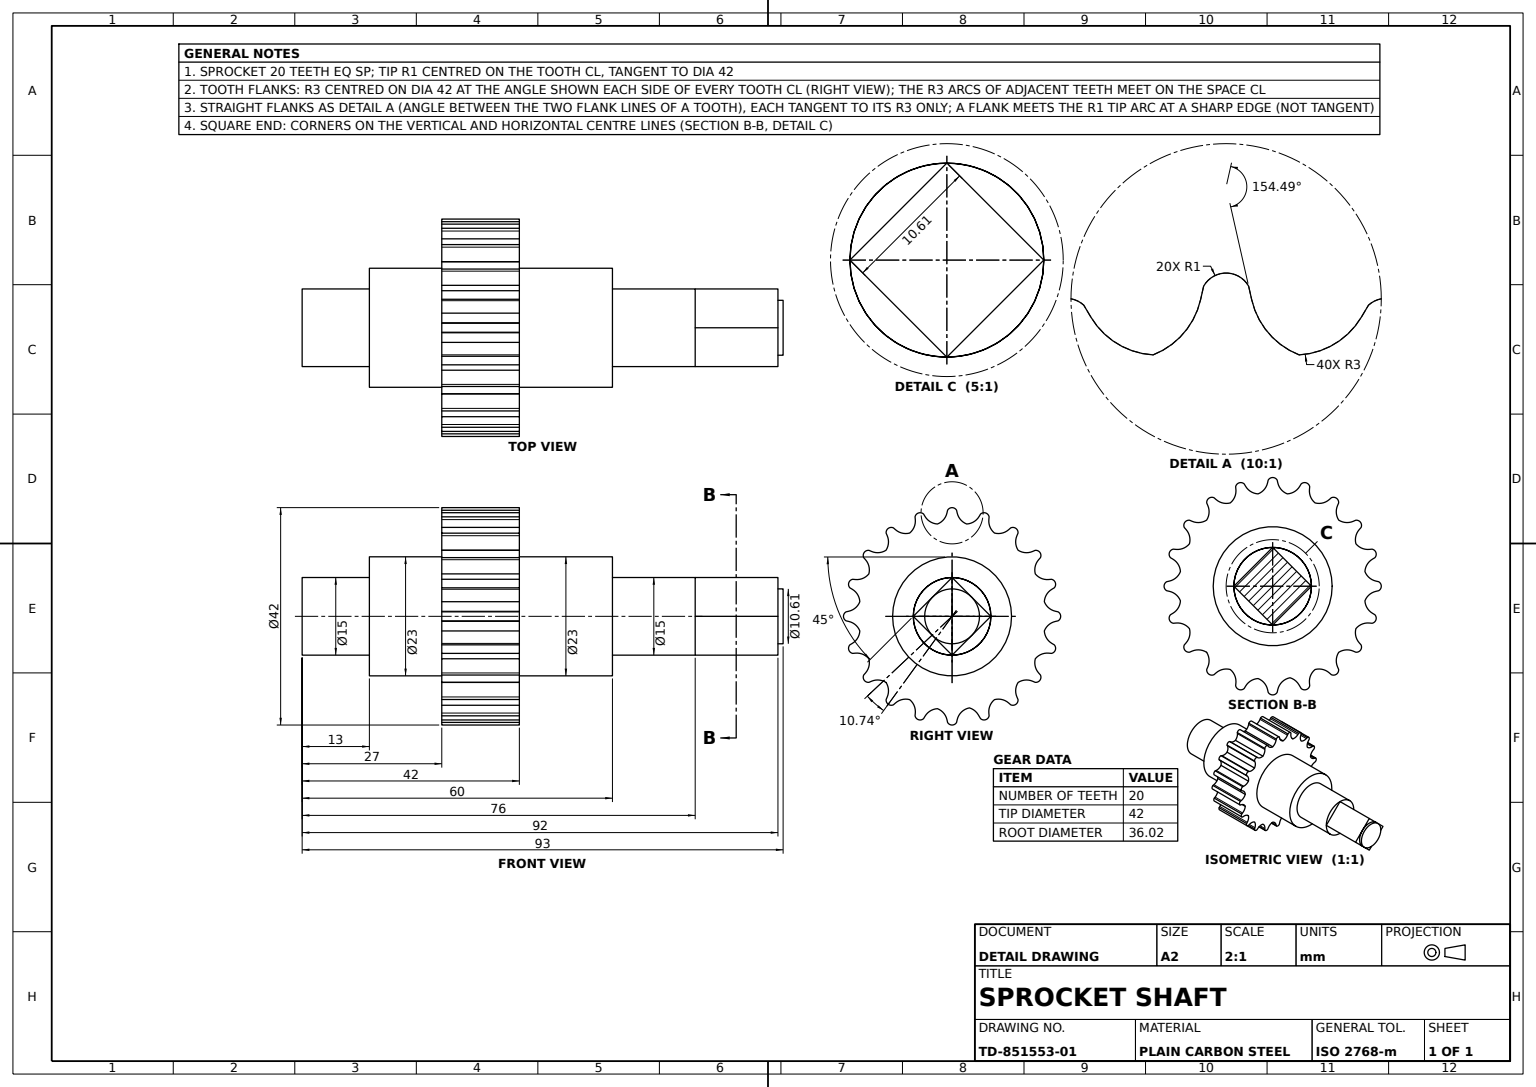
solid
v1 (12.755705,-16.18034,25.5)
v2 (12.749422,-16.068415,25.5)
e1 v1 v2 CIRCLE(AX(P(11.755705,-16.18034,25.5),D(0,0,1),D(-0.951056516,-0.309016994,0)),1)
v3 (12.755705,-16.18034,10.5)
e2 v3 v1 LINE
v4 (12.749422,-16.068415,10.5)
e3 v3 v4 CIRCLE(AX(P(11.755705,-16.18034,10.5),D(0,0,1),D(-0.951056516,-0.309016994,0)),1)
e4 v4 v2 LINE
face CYL(AX(P(11.755705,-16.18034,10.5),D(0,0,1),D(1,0,0)),1) [-e1 -e2 e3 e4]
v5 (-11.5,0,-7.5)
v6 (11.5,0,-7.5)
e5 v5 v6 CIRCLE(AX(P(0,0,-7.5),D(0,0,-1),D(-1,0,0)),11.5)
e6 v6 v5 CIRCLE(AX(P(0,0,-7.5),D(0,0,-1),D(-1,0,0)),11.5)
v7 (-7.5,0,-7.5)
v8 (7.5,0,-7.5)
e7 v7 v8 CIRCLE(AX(P(0,0,-7.5),D(0,0,-1),D(-1,0,0)),7.5)
e8 v8 v7 CIRCLE(AX(P(0,0,-7.5),D(0,0,-1),D(-1,0,0)),7.5)
face PLANE(AX(P(0,7.5,-7.5),D(0,0,-1),D(-1,0,0))) [e5 e6] [-e7 -e8]
v9 (3.75,3.75,-39.5)
v10 (5.303301,0,-39.5)
e9 v9 v10 CIRCLE(AX(P(0,0,-39.5),D(0,0,-1),D(-1,0,0)),5.303301)
v11 (7.5,0,-39.5)
e10 v9 v11 LINE
v12 (3.75,-3.75,-39.5)
e11 v11 v12 LINE
e12 v10 v12 CIRCLE(AX(P(0,0,-39.5),D(0,0,-1),D(-1,0,0)),5.303301)
face PLANE(AX(P(0,0,-39.5),D(0,0,-1),D(-1,0,0))) [-e9 e10 e11 -e12]
v13 (-16.090715,8.198629,10.5)
v14 (-16.736721,10.938339,10.5)
e13 v13 v14 CIRCLE(AX(P(-18.992374,8.960454,10.5),D(0,0,1),D(-1,0,0)),3)
v15 (-16.090715,8.198629,25.5)
e14 v15 v13 LINE
v16 (-16.736721,10.938339,25.5)
e15 v16 v15 CIRCLE(AX(P(-18.992374,8.960454,25.5),D(0,0,-1),D(1,0,0)),3)
e16 v14 v16 LINE
face CYL(AX(P(-18.992374,8.960454,0),D(0,0,-1),D(-1,0,0)),3) rev [-e13 -e14 -e15 -e16]
v17 (-17.090834,-11.342183,25.5)
v18 (-16.068415,-12.749422,25.5)
e17 v17 v18 CIRCLE(AX(P(-16.18034,-11.755705,25.5),D(0,0,1),D(-0.309016994,0.951056516,0)),1)
v19 (-17.090834,-11.342183,10.5)
e18 v19 v17 LINE
v20 (-16.068415,-12.749422,10.5)
e19 v19 v20 CIRCLE(AX(P(-16.18034,-11.755705,10.5),D(0,0,1),D(-0.309016994,0.951056516,0)),1)
e20 v20 v18 LINE
face CYL(AX(P(-16.18034,-11.755705,10.5),D(0,0,1),D(1,0,0)),1) [-e17 -e18 e19 e20]
v21 (-19.2977,-5.231047,25.5)
v22 (-19.2977,-5.231047,10.5)
e21 v21 v22 LINE
v23 (-19.759276,-5.505699,10.5)
e22 v22 v23 LINE
v24 (-19.759276,-5.505699,25.5)
e23 v23 v24 LINE
e24 v21 v24 LINE
face PLANE(AX(P(-2.747228,4.616964,10.5),D(-0.511351213,0.859371827,0),D(-0.859371827,-0.511351213,0))) [e21 e22 e23 -e24]
v25 (-8.198629,-16.090715,10.5)
v26 (-10.938339,-16.736721,10.5)
e25 v25 v26 CIRCLE(AX(P(-8.960454,-18.992374,10.5),D(0,0,1),D(-1,0,0)),3)
v27 (-8.198629,-16.090715,25.5)
e26 v27 v25 LINE
v28 (-10.938339,-16.736721,25.5)
e27 v28 v27 CIRCLE(AX(P(-8.960454,-18.992374,25.5),D(0,0,-1),D(1,0,0)),3)
e28 v26 v28 LINE
face CYL(AX(P(-8.960454,-18.992374,0),D(0,0,-1),D(-1,0,0)),3) rev [-e25 -e26 -e27 -e28]
v29 (-3.75,-3.75,-39.5)
v30 (-7.5,0,-39.5)
e29 v29 v30 LINE
v31 (0,-7.5,-39.5)
e30 v31 v29 LINE
v32 (0,-7.5,-23.5)
e31 v32 v31 LINE
v33 (-7.5,0,-23.5)
e32 v32 v33 LINE
e33 v33 v30 LINE
face PLANE(AX(P(-3.75,-3.75,-23.5),D(-0.707106781,-0.707106781,0),D(0.707106781,-0.707106781,0))) [-e29 -e30 -e31 e32 e33]
v34 (0.869722,20.493543,10.5)
v35 (0.869722,20.493543,25.5)
e34 v34 v35 LINE
v36 (-0.869722,20.493543,10.5)
e35 v34 v36 CIRCLE(AX(P(0,20,10.5),D(0,0,1),D(0.951056516,-0.309016994,0)),1)
v37 (-0.869722,20.493543,25.5)
e36 v36 v37 LINE
e37 v35 v37 CIRCLE(AX(P(0,20,25.5),D(0,0,1),D(0.951056516,-0.309016994,0)),1)
face CYL(AX(P(0,20,10.5),D(0,0,1),D(1,0,0)),1) [-e34 e35 e36 -e37]
v38 (17.18034,-11.755705,10.5)
v39 (17.090834,-11.342183,10.5)
e38 v38 v39 CIRCLE(AX(P(16.18034,-11.755705,10.5),D(0,0,1),D(-0.809016994,-0.587785252,0)),1)
v40 (17.090834,-11.342183,25.5)
e39 v39 v40 LINE
v41 (17.18034,-11.755705,25.5)
e40 v41 v40 CIRCLE(AX(P(16.18034,-11.755705,25.5),D(0,0,1),D(-0.809016994,-0.587785252,0)),1)
e41 v38 v41 LINE
face CYL(AX(P(16.18034,-11.755705,10.5),D(0,0,1),D(1,0,0)),1) [e38 e39 -e40 -e41]
v42 (17.836695,2.825055,10.5)
v43 (17.836695,2.825055,25.5)
e42 v42 v43 LINE
v44 (19.2977,5.231047,10.5)
e43 v44 v42 CIRCLE(AX(P(20.831753,2.652932,10.5),D(0,0,1),D(-1,0,0)),3)
v45 (19.2977,5.231047,25.5)
e44 v45 v44 LINE
e45 v43 v45 CIRCLE(AX(P(20.831753,2.652932,25.5),D(0,0,-1),D(1,0,0)),3)
face CYL(AX(P(20.831753,2.652932,0),D(0,0,-1),D(-1,0,0)),3) rev [-e42 -e43 -e44 -e45]
v46 (-12.769664,-12.769664,25.5)
v47 (-12.537435,-15.57491,25.5)
e46 v46 v47 CIRCLE(AX(P(-15.293888,-14.390864,25.5),D(0,0,-1),D(1,0,0)),3)
v48 (-12.749422,-16.068415,25.5)
e47 v47 v48 LINE
v49 (-11.342183,-17.090834,25.5)
e48 v48 v49 CIRCLE(AX(P(-11.755705,-16.18034,25.5),D(0,0,1),D(-0.587785252,0.809016994,0)),1)
e49 v28 v49 LINE
v50 (-7.110897,-18.6869,25.5)
e50 v27 v50 CIRCLE(AX(P(-10.098331,-18.412597,25.5),D(0,0,-1),D(1,0,0)),3)
v51 (-7.160007,-19.221758,25.5)
e51 v50 v51 LINE
v52 (-5.505699,-19.759276,25.5)
e52 v51 v52 CIRCLE(AX(P(-6.18034,-19.02113,25.5),D(0,0,1),D(-0.809016994,0.587785252,0)),1)
v53 (-5.067521,-19.02288,25.5)
e53 v53 v52 LINE
v54 (-3.355095,-17.684551,25.5)
e54 v53 v54 CIRCLE(AX(P(-2.489406,-20.556933,25.5),D(0,0,-1),D(1,0,0)),3)
v55 (-0.988296,-19.969686,25.5)
e55 v54 v55 CIRCLE(AX(P(-3.914278,-20.631976,25.5),D(0,0,-1),D(1,0,0)),3)
v56 (-0.869722,-20.493543,25.5)
e56 v55 v56 LINE
v57 (0.869722,-20.493543,25.5)
e57 v56 v57 CIRCLE(AX(P(0,-20,25.5),D(0,0,1),D(-0.951056516,0.309016994,0)),1)
v58 (0.988296,-19.969686,25.5)
e58 v58 v57 LINE
v59 (2.825055,-17.836695,25.5)
e59 v58 v59 CIRCLE(AX(P(3.914278,-20.631976,25.5),D(0,0,-1),D(1,0,0)),3)
v60 (5.231047,-19.2977,25.5)
e60 v59 v60 CIRCLE(AX(P(2.652932,-20.831753,25.5),D(0,0,-1),D(1,0,0)),3)
v61 (5.505699,-19.759276,25.5)
e61 v60 v61 LINE
v62 (7.160007,-19.221758,25.5)
e62 v61 v62 CIRCLE(AX(P(6.18034,-19.02113,25.5),D(0,0,1),D(-1,0,0)),1)
v63 (7.110897,-18.6869,25.5)
e63 v63 v62 LINE
v64 (7.098331,-18.412597,25.5)
e64 v63 v64 CIRCLE(AX(P(10.098331,-18.412597,25.5),D(0,0,-1),D(1,0,0)),3)
v65 (8.198629,-16.090715,25.5)
e65 v64 v65 CIRCLE(AX(P(10.098331,-18.412597,25.5),D(0,0,-1),D(1,0,0)),3)
v66 (10.938339,-16.736721,25.5)
e66 v65 v66 CIRCLE(AX(P(8.960454,-18.992374,25.5),D(0,0,-1),D(1,0,0)),3)
v67 (11.342183,-17.090834,25.5)
e67 v66 v67 LINE
e68 v67 v1 CIRCLE(AX(P(11.755705,-16.18034,25.5),D(0,0,1),D(-0.951056516,-0.309016994,0)),1)
v68 (12.537435,-15.57491,25.5)
e69 v68 v2 LINE
v69 (12.293888,-14.390864,25.5)
e70 v68 v69 CIRCLE(AX(P(15.293888,-14.390864,25.5),D(0,0,-1),D(1,0,0)),3)
v70 (12.769664,-12.769664,25.5)
e71 v69 v70 CIRCLE(AX(P(15.293888,-14.390864,25.5),D(0,0,-1),D(1,0,0)),3)
v71 (15.57491,-12.537435,25.5)
e72 v70 v71 CIRCLE(AX(P(14.390864,-15.293888,25.5),D(0,0,-1),D(1,0,0)),3)
v72 (16.068415,-12.749422,25.5)
e73 v71 v72 LINE
e74 v72 v41 CIRCLE(AX(P(16.18034,-11.755705,25.5),D(0,0,1),D(-0.809016994,-0.587785252,0)),1)
v73 (16.736721,-10.938339,25.5)
e75 v73 v40 LINE
v74 (15.992374,-8.960454,25.5)
e76 v73 v74 CIRCLE(AX(P(18.992374,-8.960454,25.5),D(0,0,-1),D(1,0,0)),3)
v75 (16.090715,-8.198629,25.5)
e77 v74 v75 CIRCLE(AX(P(18.992374,-8.960454,25.5),D(0,0,-1),D(1,0,0)),3)
v76 (18.6869,-7.110897,25.5)
e78 v75 v76 CIRCLE(AX(P(18.412597,-10.098331,25.5),D(0,0,-1),D(1,0,0)),3)
v77 (19.221758,-7.160007,25.5)
e79 v76 v77 LINE
v78 (20.02113,-6.18034,25.5)
e80 v77 v78 CIRCLE(AX(P(19.02113,-6.18034,25.5),D(0,0,1),D(-0.587785252,-0.809016994,0)),1)
v79 (19.759276,-5.505699,25.5)
e81 v78 v79 CIRCLE(AX(P(19.02113,-6.18034,25.5),D(0,0,1),D(-0.587785252,-0.809016994,0)),1)
v80 (19.2977,-5.231047,25.5)
e82 v80 v79 LINE
v81 (17.836695,-2.825055,25.5)
e83 v80 v81 CIRCLE(AX(P(20.831753,-2.652932,25.5),D(0,0,-1),D(1,0,0)),3)
v82 (19.969686,-0.988296,25.5)
e84 v81 v82 CIRCLE(AX(P(20.631976,-3.914278,25.5),D(0,0,-1),D(1,0,0)),3)
v83 (20.493543,-0.869722,25.5)
e85 v82 v83 LINE
v84 (21,0,25.5)
e86 v83 v84 CIRCLE(AX(P(20,0,25.5),D(0,0,1),D(-0.309016994,-0.951056516,0)),1)
v85 (20.493543,0.869722,25.5)
e87 v84 v85 CIRCLE(AX(P(20,0,25.5),D(0,0,1),D(-0.309016994,-0.951056516,0)),1)
v86 (19.969686,0.988296,25.5)
e88 v86 v85 LINE
e89 v86 v43 CIRCLE(AX(P(20.631976,3.914278,25.5),D(0,0,-1),D(1,0,0)),3)
v87 (19.759276,5.505699,25.5)
e90 v45 v87 LINE
v88 (20.02113,6.18034,25.5)
e91 v87 v88 CIRCLE(AX(P(19.02113,6.18034,25.5),D(0,0,1),D(0,-1,0)),1)
v89 (19.221758,7.160007,25.5)
e92 v88 v89 CIRCLE(AX(P(19.02113,6.18034,25.5),D(0,0,1),D(0,-1,0)),1)
v90 (18.6869,7.110897,25.5)
e93 v90 v89 LINE
v91 (16.090715,8.198629,25.5)
e94 v90 v91 CIRCLE(AX(P(18.412597,10.098331,25.5),D(0,0,-1),D(1,0,0)),3)
v92 (15.992374,8.960454,25.5)
e95 v91 v92 CIRCLE(AX(P(18.992374,8.960454,25.5),D(0,0,-1),D(1,0,0)),3)
v93 (16.736721,10.938339,25.5)
e96 v92 v93 CIRCLE(AX(P(18.992374,8.960454,25.5),D(0,0,-1),D(1,0,0)),3)
v94 (17.090834,11.342183,25.5)
e97 v93 v94 LINE
v95 (17.18034,11.755705,25.5)
e98 v94 v95 CIRCLE(AX(P(16.18034,11.755705,25.5),D(0,0,1),D(0.309016994,-0.951056516,0)),1)
v96 (16.068415,12.749422,25.5)
e99 v95 v96 CIRCLE(AX(P(16.18034,11.755705,25.5),D(0,0,1),D(0.309016994,-0.951056516,0)),1)
v97 (15.57491,12.537435,25.5)
e100 v97 v96 LINE
v98 (12.769664,12.769664,25.5)
e101 v97 v98 CIRCLE(AX(P(14.390864,15.293888,25.5),D(0,0,-1),D(1,0,0)),3)
v99 (12.293888,14.390864,25.5)
e102 v98 v99 CIRCLE(AX(P(15.293888,14.390864,25.5),D(0,0,-1),D(1,0,0)),3)
v100 (12.537435,15.57491,25.5)
e103 v99 v100 CIRCLE(AX(P(15.293888,14.390864,25.5),D(0,0,-1),D(1,0,0)),3)
v101 (12.749422,16.068415,25.5)
e104 v100 v101 LINE
v102 (12.755705,16.18034,25.5)
e105 v101 v102 CIRCLE(AX(P(11.755705,16.18034,25.5),D(0,0,1),D(0.587785252,-0.809016994,0)),1)
v103 (11.342183,17.090834,25.5)
e106 v102 v103 CIRCLE(AX(P(11.755705,16.18034,25.5),D(0,0,1),D(0.587785252,-0.809016994,0)),1)
v104 (10.938339,16.736721,25.5)
e107 v104 v103 LINE
v105 (8.198629,16.090715,25.5)
e108 v104 v105 CIRCLE(AX(P(8.960454,18.992374,25.5),D(0,0,-1),D(1,0,0)),3)
v106 (7.098331,18.412597,25.5)
e109 v105 v106 CIRCLE(AX(P(10.098331,18.412597,25.5),D(0,0,-1),D(1,0,0)),3)
v107 (7.110897,18.6869,25.5)
e110 v106 v107 CIRCLE(AX(P(10.098331,18.412597,25.5),D(0,0,-1),D(1,0,0)),3)
v108 (7.160007,19.221758,25.5)
e111 v107 v108 LINE
v109 (5.505699,19.759276,25.5)
e112 v108 v109 CIRCLE(AX(P(6.18034,19.02113,25.5),D(0,0,1),D(0.809016994,-0.587785252,0)),1)
v110 (5.231047,19.2977,25.5)
e113 v110 v109 LINE
v111 (2.825055,17.836695,25.5)
e114 v110 v111 CIRCLE(AX(P(2.652932,20.831753,25.5),D(0,0,-1),D(1,0,0)),3)
v112 (0.988296,19.969686,25.5)
e115 v111 v112 CIRCLE(AX(P(3.914278,20.631976,25.5),D(0,0,-1),D(1,0,0)),3)
e116 v112 v35 LINE
v113 (-0.988296,19.969686,25.5)
e117 v113 v37 LINE
v114 (-2.825055,17.836695,25.5)
e118 v113 v114 CIRCLE(AX(P(-3.914278,20.631976,25.5),D(0,0,-1),D(1,0,0)),3)
v115 (-5.231047,19.2977,25.5)
e119 v114 v115 CIRCLE(AX(P(-2.652932,20.831753,25.5),D(0,0,-1),D(1,0,0)),3)
v116 (-5.505699,19.759276,25.5)
e120 v115 v116 LINE
v117 (-7.160007,19.221758,25.5)
e121 v116 v117 CIRCLE(AX(P(-6.18034,19.02113,25.5),D(0,0,1),D(1,0,0)),1)
v118 (-7.110897,18.6869,25.5)
e122 v118 v117 LINE
v119 (-8.198629,16.090715,25.5)
e123 v118 v119 CIRCLE(AX(P(-10.098331,18.412597,25.5),D(0,0,-1),D(1,0,0)),3)
v120 (-10.938339,16.736721,25.5)
e124 v119 v120 CIRCLE(AX(P(-8.960454,18.992374,25.5),D(0,0,-1),D(1,0,0)),3)
v121 (-11.342183,17.090834,25.5)
e125 v120 v121 LINE
v122 (-12.749422,16.068415,25.5)
e126 v121 v122 CIRCLE(AX(P(-11.755705,16.18034,25.5),D(0,0,1),D(0.951056516,0.309016994,0)),1)
v123 (-12.537435,15.57491,25.5)
e127 v123 v122 LINE
v124 (-12.769664,12.769664,25.5)
e128 v123 v124 CIRCLE(AX(P(-15.293888,14.390864,25.5),D(0,0,-1),D(1,0,0)),3)
v125 (-15.57491,12.537435,25.5)
e129 v124 v125 CIRCLE(AX(P(-14.390864,15.293888,25.5),D(0,0,-1),D(1,0,0)),3)
v126 (-16.068415,12.749422,25.5)
e130 v125 v126 LINE
v127 (-17.090834,11.342183,25.5)
e131 v126 v127 CIRCLE(AX(P(-16.18034,11.755705,25.5),D(0,0,1),D(0.809016994,0.587785252,0)),1)
e132 v16 v127 LINE
v128 (-18.6869,7.110897,25.5)
e133 v15 v128 CIRCLE(AX(P(-18.412597,10.098331,25.5),D(0,0,-1),D(1,0,0)),3)
v129 (-19.221758,7.160007,25.5)
e134 v128 v129 LINE
v130 (-19.759276,5.505699,25.5)
e135 v129 v130 CIRCLE(AX(P(-19.02113,6.18034,25.5),D(0,0,1),D(0.587785252,0.809016994,0)),1)
v131 (-19.2977,5.231047,25.5)
e136 v131 v130 LINE
v132 (-17.836695,2.825055,25.5)
e137 v131 v132 CIRCLE(AX(P(-20.831753,2.652932,25.5),D(0,0,-1),D(1,0,0)),3)
v133 (-19.969686,0.988296,25.5)
e138 v132 v133 CIRCLE(AX(P(-20.631976,3.914278,25.5),D(0,0,-1),D(1,0,0)),3)
v134 (-20.493543,0.869722,25.5)
e139 v133 v134 LINE
v135 (-20.493543,-0.869722,25.5)
e140 v134 v135 CIRCLE(AX(P(-20,0,25.5),D(0,0,1),D(0.309016994,0.951056516,0)),1)
v136 (-19.969686,-0.988296,25.5)
e141 v136 v135 LINE
v137 (-17.836695,-2.825055,25.5)
e142 v136 v137 CIRCLE(AX(P(-20.631976,-3.914278,25.5),D(0,0,-1),D(1,0,0)),3)
e143 v137 v21 CIRCLE(AX(P(-20.831753,-2.652932,25.5),D(0,0,-1),D(1,0,0)),3)
v138 (-19.221758,-7.160007,25.5)
e144 v24 v138 CIRCLE(AX(P(-19.02113,-6.18034,25.5),D(0,0,1),D(0,1,0)),1)
v139 (-18.6869,-7.110897,25.5)
e145 v139 v138 LINE
v140 (-16.090715,-8.198629,25.5)
e146 v139 v140 CIRCLE(AX(P(-18.412597,-10.098331,25.5),D(0,0,-1),D(1,0,0)),3)
v141 (-16.736721,-10.938339,25.5)
e147 v140 v141 CIRCLE(AX(P(-18.992374,-8.960454,25.5),D(0,0,-1),D(1,0,0)),3)
e148 v141 v17 LINE
v142 (-15.57491,-12.537435,25.5)
e149 v142 v18 LINE
e150 v142 v46 CIRCLE(AX(P(-14.390864,-15.293888,25.5),D(0,0,-1),D(1,0,0)),3)
v143 (11.5,0,25.5)
v144 (-11.5,0,25.5)
e151 v143 v144 CIRCLE(AX(P(0,0,25.5),D(0,0,-1),D(-1,0,0)),11.5)
e152 v144 v143 CIRCLE(AX(P(0,0,25.5),D(0,0,-1),D(-1,0,0)),11.5)
face PLANE(AX(P(0,18,25.5),D(0,0,1),D(1,0,0))) [e46 e47 e48 -e49 e27 e50 e51 e52 -e53 e54 e55 e56 e57 -e58 e59 e60 e61 e62 -e63 e64 e65 e66 e67 e68 e1 -e69 e70 e71 e72 e73 e74 e40 -e75 e76 e77 e78 e79 e80 e81 -e82 e83 e84 e85 e86 e87 -e88 e89 e45 e90 e91 e92 -e93 e94 e95 e96 e97 e98 e99 -e100 e101 e102 e103 e104 e105 e106 -e107 e108 e109 e110 e111 e112 -e113 e114 e115 e116 e37 -e117 e118 e119 e120 e121 -e122 e123 e124 e125 e126 -e127 e128 e129 e130 e131 -e132 e15 e133 e134 e135 -e136 e137 e138 e139 e140 -e141 e142 e143 e24 e144 -e145 e146 e147 e148 e17 -e149 e150] [e151 e152]
v145 (21,0,10.5)
e153 v145 v84 LINE
v146 (20.493543,0.869722,10.5)
e154 v145 v146 CIRCLE(AX(P(20,0,10.5),D(0,0,1),D(-0.309016994,-0.951056516,0)),1)
e155 v146 v85 LINE
face CYL(AX(P(20,0,10.5),D(0,0,1),D(1,0,0)),1) [-e87 -e153 e154 e155]
v147 (-20.493543,-0.869722,10.5)
e156 v147 v135 LINE
v148 (-20.493543,0.869722,10.5)
e157 v148 v134 LINE
e158 v148 v147 CIRCLE(AX(P(-20,0,10.5),D(0,0,1),D(0.309016994,0.951056516,0)),1)
face CYL(AX(P(-20,0,10.5),D(0,0,1),D(1,0,0)),1) [e156 -e140 -e157 e158]
v149 (-15.57491,12.537435,10.5)
e159 v125 v149 LINE
v150 (-16.068415,12.749422,10.5)
e160 v149 v150 LINE
e161 v150 v126 LINE
face PLANE(AX(P(2.120423,4.936338,10.5),D(0.39468171,0.918817908,0),D(-0.918817908,0.39468171,0))) [e159 e160 e161 -e130]
v151 (-0.988296,-19.969686,10.5)
v152 (-3.355095,-17.684551,10.5)
e162 v151 v152 CIRCLE(AX(P(-3.914278,-20.631976,10.5),D(0,0,1),D(-1,0,0)),3)
e163 v55 v151 LINE
e164 v152 v54 LINE
face CYL(AX(P(-3.914278,-20.631976,0),D(0,0,-1),D(-1,0,0)),3) rev [-e162 -e163 -e55 -e164]
v153 (16.068415,-12.749422,10.5)
e165 v153 v38 CIRCLE(AX(P(16.18034,-11.755705,10.5),D(0,0,1),D(-0.809016994,-0.587785252,0)),1)
e166 v153 v72 LINE
face CYL(AX(P(16.18034,-11.755705,10.5),D(0,0,1),D(1,0,0)),1) [e165 e41 -e74 -e166]
v154 (-12.537435,-15.57491,10.5)
v155 (-12.749422,-16.068415,10.5)
e167 v154 v155 LINE
e168 v155 v48 LINE
e169 v47 v154 LINE
face PLANE(AX(P(-4.936338,2.120423,10.5),D(-0.918817908,0.39468171,0),D(-0.39468171,-0.918817908,0))) [e167 e168 -e47 e169]
v156 (15.992374,8.960454,10.5)
e170 v92 v156 LINE
v157 (16.736721,10.938339,10.5)
e171 v157 v156 CIRCLE(AX(P(18.992374,8.960454,10.5),D(0,0,1),D(-1,0,0)),3)
e172 v93 v157 LINE
face CYL(AX(P(18.992374,8.960454,0),D(0,0,-1),D(-1,0,0)),3) rev [-e96 e170 -e171 -e172]
v158 (-16.736721,-10.938339,10.5)
e173 v141 v158 LINE
e174 v158 v19 LINE
face PLANE(AX(P(-4.03949,3.542054,10.5),D(-0.751884403,0.659294961,0),D(-0.659294961,-0.751884403,0))) [e18 -e148 e173 e174]
v159 (-7.110897,18.6869,10.5)
v160 (-7.160007,19.221758,10.5)
e175 v159 v160 LINE
e176 v159 v118 LINE
e177 v160 v117 LINE
face PLANE(AX(P(-5.349983,-0.491229,10.5),D(0.995811114,0.091434264,0),D(-0.091434264,0.995811114,0))) rev [-e175 e176 e122 -e177]
v161 (-11.5,0,10.5)
v162 (11.5,0,10.5)
e178 v161 v162 CIRCLE(AX(P(0,0,10.5),D(0,0,-1),D(-1,0,0)),11.5)
e179 v162 v161 CIRCLE(AX(P(0,0,10.5),D(0,0,-1),D(-1,0,0)),11.5)
v163 (-5.067521,-19.02288,10.5)
e180 v152 v163 CIRCLE(AX(P(-2.489406,-20.556933,10.5),D(0,0,1),D(-1,0,0)),3)
v164 (-5.505699,-19.759276,10.5)
e181 v163 v164 LINE
v165 (-7.160007,-19.221758,10.5)
e182 v165 v164 CIRCLE(AX(P(-6.18034,-19.02113,10.5),D(0,0,1),D(-0.809016994,0.587785252,0)),1)
v166 (-7.110897,-18.6869,10.5)
e183 v166 v165 LINE
e184 v166 v25 CIRCLE(AX(P(-10.098331,-18.412597,10.5),D(0,0,1),D(-1,0,0)),3)
v167 (-11.342183,-17.090834,10.5)
e185 v26 v167 LINE
e186 v155 v167 CIRCLE(AX(P(-11.755705,-16.18034,10.5),D(0,0,1),D(-0.587785252,0.809016994,0)),1)
v168 (-12.769664,-12.769664,10.5)
e187 v154 v168 CIRCLE(AX(P(-15.293888,-14.390864,10.5),D(0,0,1),D(-1,0,0)),3)
v169 (-15.57491,-12.537435,10.5)
e188 v168 v169 CIRCLE(AX(P(-14.390864,-15.293888,10.5),D(0,0,1),D(-1,0,0)),3)
e189 v169 v20 LINE
v170 (-16.090715,-8.198629,10.5)
e190 v158 v170 CIRCLE(AX(P(-18.992374,-8.960454,10.5),D(0,0,1),D(-1,0,0)),3)
v171 (-18.6869,-7.110897,10.5)
e191 v170 v171 CIRCLE(AX(P(-18.412597,-10.098331,10.5),D(0,0,1),D(-1,0,0)),3)
v172 (-19.221758,-7.160007,10.5)
e192 v171 v172 LINE
e193 v23 v172 CIRCLE(AX(P(-19.02113,-6.18034,10.5),D(0,0,1),D(0,1,0)),1)
v173 (-17.836695,-2.825055,10.5)
e194 v22 v173 CIRCLE(AX(P(-20.831753,-2.652932,10.5),D(0,0,1),D(-1,0,0)),3)
v174 (-19.969686,-0.988296,10.5)
e195 v173 v174 CIRCLE(AX(P(-20.631976,-3.914278,10.5),D(0,0,1),D(-1,0,0)),3)
e196 v174 v147 LINE
v175 (-19.969686,0.988296,10.5)
e197 v175 v148 LINE
v176 (-17.836695,2.825055,10.5)
e198 v175 v176 CIRCLE(AX(P(-20.631976,3.914278,10.5),D(0,0,1),D(-1,0,0)),3)
v177 (-19.2977,5.231047,10.5)
e199 v176 v177 CIRCLE(AX(P(-20.831753,2.652932,10.5),D(0,0,1),D(-1,0,0)),3)
v178 (-19.759276,5.505699,10.5)
e200 v177 v178 LINE
v179 (-19.221758,7.160007,10.5)
e201 v179 v178 CIRCLE(AX(P(-19.02113,6.18034,10.5),D(0,0,1),D(0.587785252,0.809016994,0)),1)
v180 (-18.6869,7.110897,10.5)
e202 v180 v179 LINE
e203 v180 v13 CIRCLE(AX(P(-18.412597,10.098331,10.5),D(0,0,1),D(-1,0,0)),3)
v181 (-17.090834,11.342183,10.5)
e204 v14 v181 LINE
e205 v150 v181 CIRCLE(AX(P(-16.18034,11.755705,10.5),D(0,0,1),D(0.809016994,0.587785252,0)),1)
v182 (-12.769664,12.769664,10.5)
e206 v149 v182 CIRCLE(AX(P(-14.390864,15.293888,10.5),D(0,0,1),D(-1,0,0)),3)
v183 (-12.537435,15.57491,10.5)
e207 v182 v183 CIRCLE(AX(P(-15.293888,14.390864,10.5),D(0,0,1),D(-1,0,0)),3)
v184 (-12.749422,16.068415,10.5)
e208 v183 v184 LINE
v185 (-11.342183,17.090834,10.5)
e209 v185 v184 CIRCLE(AX(P(-11.755705,16.18034,10.5),D(0,0,1),D(0.951056516,0.309016994,0)),1)
v186 (-10.938339,16.736721,10.5)
e210 v186 v185 LINE
v187 (-8.198629,16.090715,10.5)
e211 v186 v187 CIRCLE(AX(P(-8.960454,18.992374,10.5),D(0,0,1),D(-1,0,0)),3)
e212 v187 v159 CIRCLE(AX(P(-10.098331,18.412597,10.5),D(0,0,1),D(-1,0,0)),3)
v188 (-5.505699,19.759276,10.5)
e213 v188 v160 CIRCLE(AX(P(-6.18034,19.02113,10.5),D(0,0,1),D(1,0,0)),1)
v189 (-5.231047,19.2977,10.5)
e214 v189 v188 LINE
v190 (-2.825055,17.836695,10.5)
e215 v189 v190 CIRCLE(AX(P(-2.652932,20.831753,10.5),D(0,0,1),D(-1,0,0)),3)
v191 (-0.988296,19.969686,10.5)
e216 v190 v191 CIRCLE(AX(P(-3.914278,20.631976,10.5),D(0,0,1),D(-1,0,0)),3)
e217 v191 v36 LINE
v192 (0.988296,19.969686,10.5)
e218 v192 v34 LINE
v193 (2.825055,17.836695,10.5)
e219 v192 v193 CIRCLE(AX(P(3.914278,20.631976,10.5),D(0,0,1),D(-1,0,0)),3)
v194 (5.231047,19.2977,10.5)
e220 v193 v194 CIRCLE(AX(P(2.652932,20.831753,10.5),D(0,0,1),D(-1,0,0)),3)
v195 (5.505699,19.759276,10.5)
e221 v194 v195 LINE
v196 (7.160007,19.221758,10.5)
e222 v196 v195 CIRCLE(AX(P(6.18034,19.02113,10.5),D(0,0,1),D(0.809016994,-0.587785252,0)),1)
v197 (7.110897,18.6869,10.5)
e223 v197 v196 LINE
v198 (7.098331,18.412597,10.5)
e224 v197 v198 CIRCLE(AX(P(10.098331,18.412597,10.5),D(0,0,1),D(-1,0,0)),3)
v199 (8.198629,16.090715,10.5)
e225 v198 v199 CIRCLE(AX(P(10.098331,18.412597,10.5),D(0,0,1),D(-1,0,0)),3)
v200 (10.938339,16.736721,10.5)
e226 v199 v200 CIRCLE(AX(P(8.960454,18.992374,10.5),D(0,0,1),D(-1,0,0)),3)
v201 (11.342183,17.090834,10.5)
e227 v200 v201 LINE
v202 (12.755705,16.18034,10.5)
e228 v202 v201 CIRCLE(AX(P(11.755705,16.18034,10.5),D(0,0,1),D(0.587785252,-0.809016994,0)),1)
v203 (12.749422,16.068415,10.5)
e229 v203 v202 CIRCLE(AX(P(11.755705,16.18034,10.5),D(0,0,1),D(0.587785252,-0.809016994,0)),1)
v204 (12.537435,15.57491,10.5)
e230 v204 v203 LINE
v205 (12.293888,14.390864,10.5)
e231 v204 v205 CIRCLE(AX(P(15.293888,14.390864,10.5),D(0,0,1),D(-1,0,0)),3)
v206 (12.769664,12.769664,10.5)
e232 v205 v206 CIRCLE(AX(P(15.293888,14.390864,10.5),D(0,0,1),D(-1,0,0)),3)
v207 (15.57491,12.537435,10.5)
e233 v206 v207 CIRCLE(AX(P(14.390864,15.293888,10.5),D(0,0,1),D(-1,0,0)),3)
v208 (16.068415,12.749422,10.5)
e234 v207 v208 LINE
v209 (17.18034,11.755705,10.5)
e235 v209 v208 CIRCLE(AX(P(16.18034,11.755705,10.5),D(0,0,1),D(0.309016994,-0.951056516,0)),1)
v210 (17.090834,11.342183,10.5)
e236 v210 v209 CIRCLE(AX(P(16.18034,11.755705,10.5),D(0,0,1),D(0.309016994,-0.951056516,0)),1)
e237 v157 v210 LINE
v211 (16.090715,8.198629,10.5)
e238 v156 v211 CIRCLE(AX(P(18.992374,8.960454,10.5),D(0,0,1),D(-1,0,0)),3)
v212 (18.6869,7.110897,10.5)
e239 v211 v212 CIRCLE(AX(P(18.412597,10.098331,10.5),D(0,0,1),D(-1,0,0)),3)
v213 (19.221758,7.160007,10.5)
e240 v212 v213 LINE
v214 (20.02113,6.18034,10.5)
e241 v214 v213 CIRCLE(AX(P(19.02113,6.18034,10.5),D(0,0,1),D(0,-1,0)),1)
v215 (19.759276,5.505699,10.5)
e242 v215 v214 CIRCLE(AX(P(19.02113,6.18034,10.5),D(0,0,1),D(0,-1,0)),1)
e243 v44 v215 LINE
v216 (19.969686,0.988296,10.5)
e244 v42 v216 CIRCLE(AX(P(20.631976,3.914278,10.5),D(0,0,1),D(-1,0,0)),3)
e245 v216 v146 LINE
v217 (20.493543,-0.869722,10.5)
e246 v217 v145 CIRCLE(AX(P(20,0,10.5),D(0,0,1),D(-0.309016994,-0.951056516,0)),1)
v218 (19.969686,-0.988296,10.5)
e247 v218 v217 LINE
v219 (17.836695,-2.825055,10.5)
e248 v218 v219 CIRCLE(AX(P(20.631976,-3.914278,10.5),D(0,0,1),D(-1,0,0)),3)
v220 (19.2977,-5.231047,10.5)
e249 v219 v220 CIRCLE(AX(P(20.831753,-2.652932,10.5),D(0,0,1),D(-1,0,0)),3)
v221 (19.759276,-5.505699,10.5)
e250 v220 v221 LINE
v222 (20.02113,-6.18034,10.5)
e251 v222 v221 CIRCLE(AX(P(19.02113,-6.18034,10.5),D(0,0,1),D(-0.587785252,-0.809016994,0)),1)
v223 (19.221758,-7.160007,10.5)
e252 v223 v222 CIRCLE(AX(P(19.02113,-6.18034,10.5),D(0,0,1),D(-0.587785252,-0.809016994,0)),1)
v224 (18.6869,-7.110897,10.5)
e253 v224 v223 LINE
v225 (16.090715,-8.198629,10.5)
e254 v224 v225 CIRCLE(AX(P(18.412597,-10.098331,10.5),D(0,0,1),D(-1,0,0)),3)
v226 (15.992374,-8.960454,10.5)
e255 v225 v226 CIRCLE(AX(P(18.992374,-8.960454,10.5),D(0,0,1),D(-1,0,0)),3)
v227 (16.736721,-10.938339,10.5)
e256 v226 v227 CIRCLE(AX(P(18.992374,-8.960454,10.5),D(0,0,1),D(-1,0,0)),3)
e257 v227 v39 LINE
v228 (15.57491,-12.537435,10.5)
e258 v228 v153 LINE
v229 (12.769664,-12.769664,10.5)
e259 v228 v229 CIRCLE(AX(P(14.390864,-15.293888,10.5),D(0,0,1),D(-1,0,0)),3)
v230 (12.293888,-14.390864,10.5)
e260 v229 v230 CIRCLE(AX(P(15.293888,-14.390864,10.5),D(0,0,1),D(-1,0,0)),3)
v231 (12.537435,-15.57491,10.5)
e261 v230 v231 CIRCLE(AX(P(15.293888,-14.390864,10.5),D(0,0,1),D(-1,0,0)),3)
e262 v231 v4 LINE
v232 (11.342183,-17.090834,10.5)
e263 v232 v3 CIRCLE(AX(P(11.755705,-16.18034,10.5),D(0,0,1),D(-0.951056516,-0.309016994,0)),1)
v233 (10.938339,-16.736721,10.5)
e264 v233 v232 LINE
v234 (8.198629,-16.090715,10.5)
e265 v233 v234 CIRCLE(AX(P(8.960454,-18.992374,10.5),D(0,0,1),D(-1,0,0)),3)
v235 (7.098331,-18.412597,10.5)
e266 v234 v235 CIRCLE(AX(P(10.098331,-18.412597,10.5),D(0,0,1),D(-1,0,0)),3)
v236 (7.110897,-18.6869,10.5)
e267 v235 v236 CIRCLE(AX(P(10.098331,-18.412597,10.5),D(0,0,1),D(-1,0,0)),3)
v237 (7.160007,-19.221758,10.5)
e268 v236 v237 LINE
v238 (5.505699,-19.759276,10.5)
e269 v238 v237 CIRCLE(AX(P(6.18034,-19.02113,10.5),D(0,0,1),D(-1,0,0)),1)
v239 (5.231047,-19.2977,10.5)
e270 v239 v238 LINE
v240 (2.825055,-17.836695,10.5)
e271 v239 v240 CIRCLE(AX(P(2.652932,-20.831753,10.5),D(0,0,1),D(-1,0,0)),3)
v241 (0.988296,-19.969686,10.5)
e272 v240 v241 CIRCLE(AX(P(3.914278,-20.631976,10.5),D(0,0,1),D(-1,0,0)),3)
v242 (0.869722,-20.493543,10.5)
e273 v241 v242 LINE
v243 (-0.869722,-20.493543,10.5)
e274 v243 v242 CIRCLE(AX(P(0,-20,10.5),D(0,0,1),D(-0.951056516,0.309016994,0)),1)
e275 v151 v243 LINE
face PLANE(AX(P(0,11.5,10.5),D(0,0,-1),D(-1,0,0))) [-e178 -e179] [e162 e180 e181 -e182 -e183 e184 e25 e185 -e186 -e167 e187 e188 e189 -e19 -e174 e190 e191 e192 -e193 -e22 e194 e195 e196 -e158 -e197 e198 e199 e200 -e201 -e202 e203 e13 e204 -e205 -e160 e206 e207 e208 -e209 -e210 e211 e212 e175 -e213 -e214 e215 e216 e217 -e35 -e218 e219 e220 e221 -e222 -e223 e224 e225 e226 e227 -e228 -e229 -e230 e231 e232 e233 e234 -e235 -e236 -e237 e171 e238 e239 e240 -e241 -e242 -e243 e43 e244 e245 -e154 -e246 -e247 e248 e249 e250 -e251 -e252 -e253 e254 e255 e256 e257 -e38 -e165 -e258 e259 e260 e261 e262 -e3 -e263 -e264 e265 e266 e267 e268 -e269 -e270 e271 e272 e273 -e274 -e275]
e276 v12 v29 CIRCLE(AX(P(0,0,-39.5),D(0,0,-1),D(-1,0,0)),5.303301)
e277 v12 v31 LINE
face PLANE(AX(P(0,0,-39.5),D(0,0,-1),D(-1,0,0))) [-e276 e277 e30]
e278 v162 v6 LINE
e279 v161 v5 LINE
face CYL(AX(P(0,0,0),D(0,0,-1),D(-1,0,0)),11.5) [e178 e278 -e5 -e279]
e280 v206 v98 LINE
e281 v207 v97 LINE
face CYL(AX(P(14.390864,15.293888,0),D(0,0,-1),D(-1,0,0)),3) rev [-e233 e280 -e101 -e281]
v244 (-7.5,0,52.5)
v245 (-7.5,0,39.5)
e282 v244 v245 LINE
v246 (7.5,0,39.5)
e283 v246 v245 CIRCLE(AX(P(0,0,39.5),D(0,0,-1),D(-1,0,0)),7.5)
v247 (7.5,0,52.5)
e284 v247 v246 LINE
e285 v247 v244 CIRCLE(AX(P(0,0,52.5),D(0,0,-1),D(-1,0,0)),7.5)
face CYL(AX(P(0,0,0),D(0,0,-1),D(-1,0,0)),7.5) [e282 -e283 -e284 e285]
e286 v133 v175 LINE
e287 v132 v176 LINE
face CYL(AX(P(-20.631976,3.914278,0),D(0,0,-1),D(-1,0,0)),3) rev [-e198 -e286 -e138 e287]
v248 (0,7.5,-23.5)
v249 (0,7.5,-39.5)
e288 v248 v249 LINE
v250 (7.5,0,-23.5)
e289 v248 v250 LINE
e290 v250 v11 LINE
e291 v249 v9 LINE
face PLANE(AX(P(3.75,3.75,-23.5),D(0.707106781,0.707106781,0),D(-0.707106781,0.707106781,0))) [-e288 e289 e290 -e10 -e291]
e292 v188 v116 LINE
face CYL(AX(P(-6.18034,19.02113,10.5),D(0,0,1),D(1,0,0)),1) [-e292 e213 e177 -e121]
e293 v178 v130 LINE
e294 v177 v131 LINE
face PLANE(AX(P(-2.747228,-4.616964,10.5),D(0.511351213,0.859371827,0),D(-0.859371827,0.511351213,0))) rev [e136 -e293 -e200 e294]
e295 v236 v63 LINE
e296 v64 v235 LINE
face CYL(AX(P(10.098331,-18.412597,0),D(0,0,-1),D(-1,0,0)),3) rev [-e295 -e267 -e296 -e64]
e297 v243 v56 LINE
face PLANE(AX(P(-5.239934,-1.186049,10.5),D(-0.975327391,-0.220763405,0),D(0.220763405,-0.975327391,0))) [e275 e297 -e56 e163]
e298 v60 v239 LINE
e299 v238 v61 LINE
face PLANE(AX(P(-4.616964,-2.747228,10.5),D(-0.859371827,-0.511351213,0),D(0.511351213,-0.859371827,0))) [-e61 e298 e270 e299]
e300 v124 v182 LINE
face CYL(AX(P(-14.390864,15.293888,0),D(0,0,-1),D(-1,0,0)),3) rev [-e159 -e129 e300 -e206]
e301 v212 v90 LINE
e302 v211 v91 LINE
face CYL(AX(P(18.412597,10.098331,0),D(0,0,-1),D(-1,0,0)),3) rev [-e301 -e239 e302 -e94]
v251 (5.303301,0,-40.5)
e303 v251 v10 LINE
v252 (-5.303301,0,-39.5)
e304 v29 v252 CIRCLE(AX(P(0,0,-39.5),D(0,0,-1),D(-1,0,0)),5.303301)
v253 (-5.303301,0,-40.5)
e305 v253 v252 LINE
e306 v251 v253 CIRCLE(AX(P(0,0,-40.5),D(0,0,-1),D(-1,0,0)),5.303301)
face CYL(AX(P(0,0,-40.5),D(0,0,1),D(1,0,0)),5.303301) [e303 e12 e276 e304 -e305 -e306]
e307 v100 v204 LINE
e308 v203 v101 LINE
face PLANE(AX(P(4.936338,-2.120423,10.5),D(0.918817908,-0.39468171,0),D(0.39468171,0.918817908,0))) [e307 e230 e308 -e104]
e309 v250 v32 CIRCLE(AX(P(0,0,-23.5),D(0,0,-1),D(-1,0,0)),7.5)
e310 v8 v250 LINE
e311 v7 v33 LINE
e312 v32 v33 CIRCLE(AX(P(0,0,-23.5),D(0,0,-1),D(-1,0,0)),7.5)
face CYL(AX(P(0,0,0),D(0,0,-1),D(-1,0,0)),7.5) [-e309 -e310 e8 e311 -e312]
e313 v222 v78 LINE
e314 v223 v77 LINE
face CYL(AX(P(19.02113,-6.18034,10.5),D(0,0,1),D(1,0,0)),1) [e252 e313 -e80 -e314]
face CYL(AX(P(-20.831753,2.652932,0),D(0,0,-1),D(-1,0,0)),3) rev [-e199 -e287 -e137 -e294]
e315 v115 v189 LINE
face PLANE(AX(P(4.616964,2.747228,10.5),D(0.859371827,0.511351213,0),D(-0.511351213,0.859371827,0))) [e292 -e120 e315 e214]
e316 v217 v83 LINE
e317 v82 v218 LINE
face PLANE(AX(P(1.186049,-5.239934,10.5),D(0.220763405,-0.975327391,0),D(0.975327391,0.220763405,0))) [e316 -e85 e317 e247]
e318 v196 v108 LINE
e319 v107 v197 LINE
face PLANE(AX(P(5.349983,-0.491229,10.5),D(0.995811114,-0.091434264,0),D(0.091434264,0.995811114,0))) [e318 -e111 e319 e223]
e320 v120 v186 LINE
e321 v185 v121 LINE
face PLANE(AX(P(3.542054,4.03949,10.5),D(0.659294961,0.751884403,0),D(-0.751884403,0.659294961,0))) [-e125 e320 e210 e321]
e322 v71 v228 LINE
e323 v229 v70 LINE
face CYL(AX(P(14.390864,-15.293888,0),D(0,0,-1),D(-1,0,0)),3) rev [-e322 -e72 -e323 -e259]
e324 v137 v173 LINE
face CYL(AX(P(-20.831753,-2.652932,0),D(0,0,-1),D(-1,0,0)),3) rev [-e194 -e21 -e143 e324]
e325 v46 v168 LINE
e326 v169 v142 LINE
face CYL(AX(P(-14.390864,-15.293888,0),D(0,0,-1),D(-1,0,0)),3) rev [-e325 -e150 -e326 -e188]
face CYL(AX(P(18.992374,8.960454,0),D(0,0,-1),D(-1,0,0)),3) rev [-e302 -e238 -e170 -e95]
v254 (11.5,0,39.5)
e327 v254 v143 LINE
v255 (-11.5,0,39.5)
e328 v254 v255 CIRCLE(AX(P(0,0,39.5),D(0,0,-1),D(-1,0,0)),11.5)
e329 v255 v144 LINE
face CYL(AX(P(0,0,0),D(0,0,-1),D(-1,0,0)),11.5) [-e151 -e327 e328 e329]
e330 v244 v247 CIRCLE(AX(P(0,0,52.5),D(0,0,-1),D(-1,0,0)),7.5)
face PLANE(AX(P(0,7.5,52.5),D(0,0,1),D(1,0,0))) [-e330 -e285]
e331 v171 v139 LINE
e332 v140 v170 LINE
face CYL(AX(P(-18.412597,-10.098331,0),D(0,0,-1),D(-1,0,0)),3) rev [-e146 -e331 -e191 -e332]
e333 v114 v190 LINE
face CYL(AX(P(-2.652932,20.831753,0),D(0,0,-1),D(-1,0,0)),3) rev [-e315 -e119 e333 -e215]
e334 v50 v166 LINE
face CYL(AX(P(-10.098331,-18.412597,0),D(0,0,-1),D(-1,0,0)),3) rev [-e334 -e50 e26 -e184]
e335 v240 v59 LINE
face CYL(AX(P(2.652932,-20.831753,0),D(0,0,-1),D(-1,0,0)),3) rev [-e298 -e60 -e335 -e271]
e336 v210 v94 LINE
e337 v209 v95 LINE
face CYL(AX(P(16.18034,11.755705,10.5),D(0,0,1),D(1,0,0)),1) [-e336 e236 e337 -e98]
e338 v172 v138 LINE
face PLANE(AX(P(0.491229,-5.349983,10.5),D(-0.091434264,0.995811114,0),D(-0.995811114,-0.091434264,0))) rev [-e338 -e192 e331 e145]
e339 v250 v32 LINE
face PLANE(AX(P(0,0,-23.5),D(0,0,-1),D(-1,0,0))) [-e339 e309]
e340 v165 v51 LINE
face PLANE(AX(P(-5.349983,0.491229,10.5),D(-0.995811114,0.091434264,0),D(-0.091434264,-0.995811114,0))) [e334 e183 e340 -e51]
e341 v245 v246 CIRCLE(AX(P(0,0,39.5),D(0,0,-1),D(-1,0,0)),7.5)
face CYL(AX(P(0,0,0),D(0,0,-1),D(-1,0,0)),7.5) [-e341 -e282 e330 e284]
v256 (-3.75,3.75,-39.5)
e342 v252 v256 CIRCLE(AX(P(0,0,-39.5),D(0,0,-1),D(-1,0,0)),5.303301)
e343 v256 v9 CIRCLE(AX(P(0,0,-39.5),D(0,0,-1),D(-1,0,0)),5.303301)
e344 v253 v251 CIRCLE(AX(P(0,0,-40.5),D(0,0,-1),D(-1,0,0)),5.303301)
face CYL(AX(P(0,0,-40.5),D(0,0,1),D(1,0,0)),5.303301) [e342 e343 e9 -e303 -e344 e305]
e345 v69 v230 LINE
face CYL(AX(P(15.293888,-14.390864,0),D(0,0,-1),D(-1,0,0)),3) rev [e345 -e260 e323 -e71]
e346 v200 v104 LINE
e347 v199 v105 LINE
face CYL(AX(P(8.960454,18.992374,0),D(0,0,-1),D(-1,0,0)),3) rev [-e346 -e226 e347 -e108]
face CYL(AX(P(-18.992374,-8.960454,0),D(0,0,-1),D(-1,0,0)),3) rev [-e147 e332 -e190 -e173]
e348 v219 v81 LINE
e349 v220 v80 LINE
face CYL(AX(P(20.831753,-2.652932,0),D(0,0,-1),D(-1,0,0)),3) rev [e348 -e83 -e349 -e249]
face CYL(AX(P(20.631976,-3.914278,0),D(0,0,-1),D(-1,0,0)),3) rev [-e348 -e248 -e317 -e84]
e350 v221 v79 LINE
face CYL(AX(P(19.02113,-6.18034,10.5),D(0,0,1),D(1,0,0)),1) [-e81 -e313 e251 e350]
e351 v216 v86 LINE
face CYL(AX(P(20.631976,3.914278,0),D(0,0,-1),D(-1,0,0)),3) rev [-e351 -e244 e42 -e89]
face CYL(AX(P(-19.02113,-6.18034,10.5),D(0,0,1),D(1,0,0)),1) [-e144 -e23 e193 e338]
e352 v74 v226 LINE
e353 v225 v75 LINE
face CYL(AX(P(18.992374,-8.960454,0),D(0,0,-1),D(-1,0,0)),3) rev [-e77 e352 -e255 e353]
face CYL(AX(P(-15.293888,-14.390864,0),D(0,0,-1),D(-1,0,0)),3) rev [-e187 -e169 -e46 e325]
e354 v119 v187 LINE
face CYL(AX(P(-10.098331,18.412597,0),D(0,0,-1),D(-1,0,0)),3) rev [-e354 -e123 -e176 -e212]
e355 v227 v73 LINE
face PLANE(AX(P(4.03949,3.542054,10.5),D(-0.751884403,-0.659294961,0),D(0.659294961,-0.751884403,0))) rev [e355 e75 -e39 -e257]
e356 v164 v52 LINE
face CYL(AX(P(-6.18034,-19.02113,10.5),D(0,0,1),D(1,0,0)),1) [-e52 -e340 e182 e356]
e357 v242 v57 LINE
face CYL(AX(P(0,-20,10.5),D(0,0,1),D(1,0,0)),1) [-e297 e274 e357 -e57]
e358 v106 v198 LINE
face CYL(AX(P(10.098331,18.412597,0),D(0,0,-1),D(-1,0,0)),3) rev [-e347 -e225 -e358 -e109]
face CYL(AX(P(-8.960454,18.992374,0),D(0,0,-1),D(-1,0,0)),3) rev [e354 -e211 -e320 -e124]
e359 v181 v127 LINE
face PLANE(AX(P(-4.03949,-3.542054,10.5),D(0.751884403,0.659294961,0),D(-0.659294961,0.751884403,0))) rev [-e204 e16 e132 -e359]
face PLANE(AX(P(4.03949,-3.542054,10.5),D(0.751884403,-0.659294961,0),D(0.659294961,0.751884403,0))) [e237 e336 -e97 e172]
e360 v195 v109 LINE
face CYL(AX(P(6.18034,19.02113,10.5),D(0,0,1),D(1,0,0)),1) [e360 -e112 -e318 e222]
e361 v167 v49 LINE
face PLANE(AX(P(3.542054,-4.03949,10.5),D(-0.659294961,0.751884403,0),D(-0.751884403,-0.659294961,0))) rev [-e361 -e185 e28 e49]
e362 v99 v205 LINE
face CYL(AX(P(15.293888,14.390864,0),D(0,0,-1),D(-1,0,0)),3) rev [-e280 -e232 -e362 -e102]
e363 v241 v58 LINE
face PLANE(AX(P(5.239934,-1.186049,10.5),D(-0.975327391,0.220763405,0),D(-0.220763405,-0.975327391,0))) rev [-e273 e363 e58 -e357]
e364 v128 v180 LINE
face CYL(AX(P(-18.412597,10.098331,0),D(0,0,-1),D(-1,0,0)),3) rev [-e133 e14 -e203 -e364]
face PLANE(AX(P(-1.186049,5.239934,10.5),D(-0.220763405,0.975327391,0),D(-0.975327391,-0.220763405,0))) [e157 -e139 e286 e197]
face PLANE(AX(P(1.186049,5.239934,10.5),D(-0.220763405,-0.975327391,0),D(0.975327391,-0.220763405,0))) rev [e88 -e155 -e245 e351]
e365 v174 v136 LINE
face CYL(AX(P(-20.631976,-3.914278,0),D(0,0,-1),D(-1,0,0)),3) rev [-e195 -e324 -e142 -e365]
face CYL(AX(P(18.992374,-8.960454,0),D(0,0,-1),D(-1,0,0)),3) rev [-e76 -e355 -e256 -e352]
face PLANE(AX(P(0,0,-40.5),D(0,0,-1),D(-1,0,0))) [e344 e306]
e366 v248 v250 CIRCLE(AX(P(0,0,-23.5),D(0,0,-1),D(-1,0,0)),7.5)
e367 v33 v248 CIRCLE(AX(P(0,0,-23.5),D(0,0,-1),D(-1,0,0)),7.5)
face CYL(AX(P(0,0,0),D(0,0,-1),D(-1,0,0)),7.5) [-e366 -e367 -e311 e7 e310]
e368 v33 v248 LINE
face PLANE(AX(P(0,0,-23.5),D(0,0,-1),D(-1,0,0))) [-e368 e367]
e369 v194 v110 LINE
e370 v193 v111 LINE
face CYL(AX(P(2.652932,20.831753,0),D(0,0,-1),D(-1,0,0)),3) rev [-e114 -e369 -e220 e370]
face PLANE(AX(P(-4.616964,2.747228,10.5),D(0.859371827,-0.511351213,0),D(0.511351213,0.859371827,0))) rev [-e221 e369 e113 -e360]
e371 v112 v192 LINE
face CYL(AX(P(3.914278,20.631976,0),D(0,0,-1),D(-1,0,0)),3) rev [-e219 -e371 -e115 -e370]
face CYL(AX(P(20,0,10.5),D(0,0,1),D(1,0,0)),1) [e153 -e86 -e316 e246]
face PLANE(AX(P(3.75,-3.75,-23.5),D(0.707106781,-0.707106781,0),D(0.707106781,0.707106781,0))) [-e277 -e11 -e290 e339 e31]
e372 v231 v68 LINE
face PLANE(AX(P(4.936338,2.120423,10.5),D(-0.918817908,-0.39468171,0),D(0.39468171,-0.918817908,0))) rev [-e262 e372 e69 -e4]
face CYL(AX(P(15.293888,14.390864,0),D(0,0,-1),D(-1,0,0)),3) rev [-e103 e362 -e231 -e307]
e373 v208 v96 LINE
face CYL(AX(P(16.18034,11.755705,10.5),D(0,0,1),D(1,0,0)),1) [-e337 e235 e373 -e99]
face PLANE(AX(P(-2.120423,-4.936338,10.5),D(-0.39468171,-0.918817908,0),D(0.918817908,-0.39468171,0))) [e322 e258 e166 -e73]
e374 v76 v224 LINE
face PLANE(AX(P(-0.491229,-5.349983,10.5),D(-0.091434264,-0.995811114,0),D(0.995811114,-0.091434264,0))) [-e79 e374 e253 e314]
e375 v30 v256 LINE
face PLANE(AX(P(0,0,-39.5),D(0,0,-1),D(-1,0,0))) [e375 -e342 -e304 e29]
e376 v213 v89 LINE
face PLANE(AX(P(-0.491229,5.349983,10.5),D(0.091434264,-0.995811114,0),D(0.995811114,0.091434264,0))) rev [e301 e93 -e376 -e240]
e377 v215 v87 LINE
e378 v214 v88 LINE
face CYL(AX(P(19.02113,6.18034,10.5),D(0,0,1),D(1,0,0)),1) [-e91 -e377 e242 e378]
face CYL(AX(P(10.098331,18.412597,0),D(0,0,-1),D(-1,0,0)),3) rev [-e319 -e110 e358 -e224]
e379 v191 v113 LINE
face PLANE(AX(P(-5.239934,1.186049,10.5),D(0.975327391,-0.220763405,0),D(0.220763405,0.975327391,0))) rev [e117 -e36 -e217 e379]
e380 v66 v233 LINE
e381 v234 v65 LINE
face CYL(AX(P(8.960454,-18.992374,0),D(0,0,-1),D(-1,0,0)),3) rev [-e265 -e380 -e66 -e381]
face CYL(AX(P(3.914278,-20.631976,0),D(0,0,-1),D(-1,0,0)),3) rev [-e59 -e363 -e272 e335]
face PLANE(AX(P(0,0,-23.5),D(0,0,-1),D(-1,0,0))) [-e32 e312]
e382 v179 v129 LINE
face CYL(AX(P(-19.02113,6.18034,10.5),D(0,0,1),D(1,0,0)),1) [-e382 e201 e293 -e135]
face PLANE(AX(P(-2.120423,4.936338,10.5),D(0.39468171,-0.918817908,0),D(0.918817908,0.39468171,0))) rev [e100 -e373 -e234 e281]
face CYL(AX(P(18.412597,-10.098331,0),D(0,0,-1),D(-1,0,0)),3) rev [-e374 -e78 -e353 -e254]
face CYL(AX(P(-16.18034,11.755705,10.5),D(0,0,1),D(1,0,0)),1) [-e131 -e161 e205 e359]
e383 v232 v67 LINE
face CYL(AX(P(11.755705,-16.18034,10.5),D(0,0,1),D(1,0,0)),1) [e2 -e68 -e383 e263]
face PLANE(AX(P(0,0,-23.5),D(0,0,-1),D(-1,0,0))) [e366 -e289]
face CYL(AX(P(19.02113,6.18034,10.5),D(0,0,1),D(1,0,0)),1) [-e378 e241 e376 -e92]
face PLANE(AX(P(2.747228,4.616964,10.5),D(-0.511351213,-0.859371827,0),D(0.859371827,-0.511351213,0))) rev [-e250 e349 e82 -e350]
face CYL(AX(P(-3.914278,20.631976,0),D(0,0,-1),D(-1,0,0)),3) rev [-e118 -e379 -e216 -e333]
face PLANE(AX(P(-3.542054,-4.03949,10.5),D(-0.659294961,-0.751884403,0),D(0.751884403,-0.659294961,0))) [e383 -e67 e380 e264]
e384 v256 v249 LINE
face PLANE(AX(P(-3.75,3.75,-23.5),D(-0.707106781,0.707106781,0),D(-0.707106781,-0.707106781,0))) [-e375 -e33 e368 e288 -e384]
e385 v202 v102 LINE
face CYL(AX(P(11.755705,16.18034,10.5),D(0,0,1),D(1,0,0)),1) [e229 e385 -e105 -e308]
e386 v183 v123 LINE
face CYL(AX(P(-15.293888,14.390864,0),D(0,0,-1),D(-1,0,0)),3) rev [-e128 -e386 -e207 -e300]
face PLANE(AX(P(0.491229,5.349983,10.5),D(0.091434264,0.995811114,0),D(-0.995811114,0.091434264,0))) [e202 e382 -e134 e364]
face PLANE(AX(P(0,0,-39.5),D(0,0,-1),D(-1,0,0))) [-e343 e384 e291]
face CYL(AX(P(10.098331,-18.412597,0),D(0,0,-1),D(-1,0,0)),3) rev [e296 -e266 e381 -e65]
e387 v237 v62 LINE
face CYL(AX(P(6.18034,-19.02113,10.5),D(0,0,1),D(1,0,0)),1) [e387 -e62 -e299 e269]
face PLANE(AX(P(5.239934,1.186049,10.5),D(0.975327391,0.220763405,0),D(-0.220763405,0.975327391,0))) [e34 -e116 e371 e218]
e388 v255 v254 CIRCLE(AX(P(0,0,39.5),D(0,0,-1),D(-1,0,0)),11.5)
face CYL(AX(P(0,0,0),D(0,0,-1),D(-1,0,0)),11.5) [-e152 -e329 e388 e327]
e389 v201 v103 LINE
face CYL(AX(P(11.755705,16.18034,10.5),D(0,0,1),D(1,0,0)),1) [e389 -e106 -e385 e228]
e390 v184 v122 LINE
face PLANE(AX(P(-4.936338,-2.120423,10.5),D(0.918817908,0.39468171,0),D(-0.39468171,0.918817908,0))) rev [-e208 e386 e127 -e390]
face PLANE(AX(P(-1.186049,-5.239934,10.5),D(0.220763405,0.975327391,0),D(-0.975327391,0.220763405,0))) rev [e365 e141 -e156 -e196]
face CYL(AX(P(-11.755705,-16.18034,10.5),D(0,0,1),D(1,0,0)),1) [-e168 e186 e361 -e48]
face PLANE(AX(P(2.747228,-4.616964,10.5),D(0.511351213,-0.859371827,0),D(0.859371827,0.511351213,0))) [e44 e243 e377 -e90]
face CYL(AX(P(0,0,0),D(0,0,-1),D(-1,0,0)),11.5) [-e278 e179 e279 -e6]
face CYL(AX(P(15.293888,-14.390864,0),D(0,0,-1),D(-1,0,0)),3) rev [-e70 -e372 -e261 -e345]
e391 v163 v53 LINE
face CYL(AX(P(-2.489406,-20.556933,0),D(0,0,-1),D(-1,0,0)),3) rev [-e391 -e180 e164 -e54]
face PLANE(AX(P(0,11.5,39.5),D(0,0,1),D(1,0,0))) [e283 e341] [-e388 -e328]
face CYL(AX(P(-11.755705,16.18034,10.5),D(0,0,1),D(1,0,0)),1) [e390 -e126 -e321 e209]
face PLANE(AX(P(4.616964,-2.747228,10.5),D(-0.859371827,0.511351213,0),D(-0.511351213,-0.859371827,0))) rev [-e181 e391 e53 -e356]
face PLANE(AX(P(5.349983,0.491229,10.5),D(-0.995811114,-0.091434264,0),D(0.091434264,-0.995811114,0))) rev [e295 e63 -e387 -e268]
face PLANE(AX(P(2.120423,-4.936338,10.5),D(-0.39468171,0.918817908,0),D(-0.918817908,-0.39468171,0))) rev [-e20 -e189 e326 e149]
face PLANE(AX(P(-3.542054,4.03949,10.5),D(0.659294961,-0.751884403,0),D(0.751884403,0.659294961,0))) rev [e107 -e389 -e227 e346]
